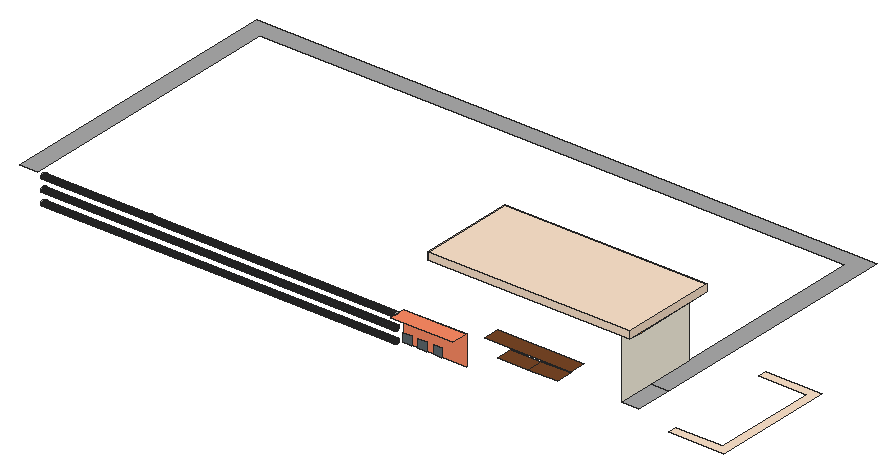
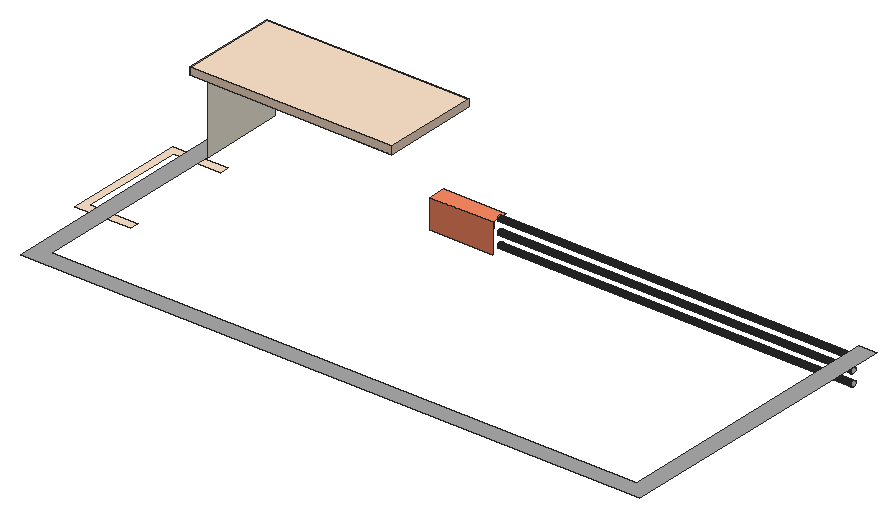
# SketchUp Ruby script. Lengths in inches.
U = 1.inch
M = Sketchup.active_model
def pt(a) = Geom::Point3d.new(a.map { |v| v * U })
def face(e, loops, mat)
  f = e.add_face(loops[0].map { |a| pt(a) })
  loops[1..].each { |l| e.add_face(l.map { |a| pt(a) }).erase! }
  f.material = f.back_material = mat if mat
  f
end
# faces: each face lists its corners as indices into pts; further lists are holes
def faces(e, pts, list, mat = nil) = list.each { |f| face(e, (f[0].is_a?(Array) ? f : [f]).map { |l| l.map { |i| pts[i] } }, mat) }
# xy, xz, yz: faces in a plane at the given z, y or x. An outline is a flat list of corners, or four numbers for a rectangle; further outlines are holes
def ring(l) = l.size == 4 ? [[l[0], l[1]], [l[2], l[1]], [l[2], l[3]], [l[0], l[3]]] : l.each_slice(2).to_a
def flat(e, list, mat, &to3) = list.each { |f| face(e, (f[0].is_a?(Array) ? f : [f]).map { |l| ring(l).map { |u, v| to3.(u, v) } }, mat) }
def xy(e, z, list, mat = nil) = flat(e, list, mat) { |x, y| [x, y, z] }
def xz(e, y, list, mat = nil) = flat(e, list, mat) { |x, z| [x, y, z] }
def yz(e, x, list, mat = nil) = flat(e, list, mat) { |y, z| [x, y, z] }
def lines(e, pts, list) = list.each { |a, b| e.add_line(pt(pts[a]), pt(pts[b])) }
# prism: a flat outline (further loops are holes) pulled along v
def prism(e, loops, v, mat = nil)
  f = face(e, loops, mat); d = Geom::Vector3d.new(v.map { |x| x * U })
  f.pushpull(f.normal.samedirection?(d) ? d.length : -d.length)
end
def box(e, o, s, mat = nil) = prism(e, [[o, [o[0] + s[0], o[1], o[2]], [o[0] + s[0], o[1] + s[1], o[2]], [o[0], o[1] + s[1], o[2]]]], [0, 0, s[2]], mat)
def at(x, y, z, deg = 0) = Geom::Transformation.translation(pt([x, y, z])) * Geom::Transformation.rotation(ORIGIN, Z_AXIS, deg.degrees)
def axes(o, x, y, z) = Geom::Transformation.new([*x, 0, *y, 0, *z, 0, *pt(o).to_a, 1])
def part(name) = M.definitions.add(name)
# library, detail: a bought-in or finely detailed component or shape, given as its bounding box
def library(name, o, s) = part(name).tap { |d| box(d.entities, o, s) }
def detail(e, o, s) = box(e.add_group.entities, o, s)
def put(e, d, t, mat = nil) = e.add_instance(d, t).tap { |i| i.material = mat if mat }
def group(e, t, mat = nil) = e.add_group.tap { |g| g.transformation = t; g.material = mat if mat }.entities
root = M.entities
M.materials.add("[Color B03]").color = [255, 140, 101]
M.materials.add("[Color C01]1").color = [255, 229, 204]
M.materials.add("[Color M03]").color = [170, 170, 170]
M.materials.add("[Formica Graystone]1").color = [255, 249, 231]
M.materials.add("[Formica Laminate Dark]").color = [50, 53, 60]
M.materials.add("[Formica Speckled Grey]").color = [94, 105, 111]
M.materials.add("[Wood Bamboo]").color = [177, 105, 43]
M.materials.add("[Wood Veneer 01]").color = [120, 70, 37]
xy(root,1017.818,[[1713.027,219.809,1866.152,219.809,1866.152,557.621,1713.027,557.621,1713.027,533.576,1844.714,533.576,1844.714,243.888,1713.027,243.888]],"[Color C01]1")
xy(root,1099.25,[[147.908,137.16,149.591,137.382,151.158,138.031,152.504,139.064,153.537,140.41,154.187,141.978,154.408,143.66,154.187,145.343,153.537,146.91,152.504,148.257,151.158,149.289,149.591,149.939,147.908,150.16,146.226,149.939,144.658,149.289,143.312,148.257,142.279,146.91,141.63,145.343,141.408,143.66,141.63,141.978,142.279,140.41,143.312,139.064,144.658,138.031,146.226,137.382]])
xy(root,1100.625,[[582.033,137.16,583.716,137.382,585.283,138.031,586.629,139.064,587.662,140.41,588.312,141.978,588.533,143.66,588.312,145.343,587.662,146.91,586.629,148.257,585.283,149.289,583.716,149.939,582.033,150.16,580.351,149.939,578.783,149.289,577.437,148.257,576.404,146.91,575.755,145.343,575.533,143.66,575.755,141.978,576.404,140.41,577.437,139.064,578.783,138.031,580.351,137.382]])
xy(root,1101.75,[[797.721,137.16,799.403,137.382,800.971,138.031,802.317,139.064,803.35,140.41,803.999,141.978,804.221,143.66,803.999,145.343,803.35,146.91,802.317,148.257,800.971,149.289,799.403,149.939,797.721,150.16,796.038,149.939,794.471,149.289,793.125,148.257,792.092,146.91,791.442,145.343,791.221,143.66,791.442,141.978,792.092,140.41,793.125,139.064,794.471,138.031,796.038,137.382],[984.137,138.709,985.819,138.93,987.387,139.58,988.733,140.613,989.766,141.959,990.416,143.527,990.637,145.209,990.416,146.891,989.766,148.459,988.733,149.805,987.387,150.838,985.819,151.487,984.137,151.709,982.455,151.487,980.887,150.838,979.541,149.805,978.508,148.459,977.859,146.891,977.637,145.209,977.859,143.527,978.508,141.959,979.541,140.613,980.887,139.58,982.455,138.93]])
xy(root,1102.645,[[1025.893,119.173,1198.268,166.042]],"[Color B03]")
xy(root,1104.303,[[341.783,137.16,343.466,137.382,345.033,138.031,346.379,139.064,347.412,140.41,348.062,141.978,348.283,143.66,348.062,145.343,347.412,146.91,347.14,147.265,336.426,147.265,336.154,146.91,335.505,145.343,335.283,143.66,335.505,141.978,336.154,140.41,337.187,139.064,338.533,138.031,340.101,137.382],[336.426,147.265,347.14,147.265,346.379,148.257,345.033,149.289,343.466,149.939,341.783,150.16,340.101,149.939,338.533,149.289,337.187,148.257]])
xy(root,1119.0625,[[1665.331,119.173,1713.027,219.809],[0,122.542,47.696,122.542,47.696,890.389,1665.331,890.389,1665.331,219.809,1713.027,219.809,1713.027,938.085,0,938.085]],"[Color M03]")
xy(root,1139.823,[[1358.015,73.861,1440.68,119.173],[1440.68,73.861,1523.345,119.173]],"[Wood Veneer 01]")
xy(root,1175.689,[[1322.149,73.861,1559.211,119.173]],"[Wood Veneer 01]")
xy(root,1305.375,[[1170.509,105.516,1168.39,105.795,1166.415,106.613,1164.719,107.914,1163.418,109.61,1162.6,111.585,1162.321,113.704,1162.6,115.823,1163.418,117.798,1164.719,119.493,1166.415,120.794,1168.39,121.612,1170.509,121.891,1172.628,121.612,1174.603,120.794,1176.298,119.493,1177.599,117.798,1178.417,115.823,1178.696,113.704,1178.417,111.585,1177.599,109.61,1176.298,107.914,1174.603,106.613,1172.628,105.795],[1198.268,119.173,1665.331,351.292],[1170.509,146.891,1168.39,147.17,1166.415,147.988,1164.719,149.289,1163.418,150.985,1162.6,152.96,1162.321,155.079,1162.6,157.198,1163.418,159.173,1164.719,160.868,1166.415,162.169,1168.39,162.987,1170.509,163.266,1172.628,162.987,1174.603,162.169,1176.298,160.868,1177.599,159.173,1178.417,157.198,1178.696,155.079,1178.417,152.96,1177.599,150.985,1176.298,149.289,1174.603,147.988,1172.628,147.17],[1170.509,209.204,1168.39,209.483,1166.415,210.301,1164.719,211.602,1163.418,213.298,1162.6,215.272,1162.321,217.391,1162.6,219.51,1163.418,221.485,1164.719,223.181,1166.415,224.482,1168.39,225.3,1170.509,225.579,1172.628,225.3,1174.603,224.482,1176.298,223.181,1177.599,221.485,1178.417,219.51,1178.696,217.391,1178.417,215.272,1177.599,213.298,1176.298,211.602,1174.603,210.301,1172.628,209.483],[1170.509,273.891,1168.39,274.17,1166.415,274.988,1164.719,276.289,1163.418,277.985,1162.6,279.96,1162.321,282.079,1162.6,284.198,1163.418,286.173,1164.719,287.868,1166.415,289.169,1168.39,289.987,1170.509,290.266,1172.628,289.987,1174.603,289.169,1176.298,287.868,1177.599,286.173,1178.417,284.198,1178.696,282.079,1178.417,279.96,1177.599,277.985,1176.298,276.289,1174.603,274.988,1172.628,274.17],
  [1170.509,317.579,1168.39,317.858,1166.415,318.676,1164.719,319.977,1163.418,321.673,1162.6,323.647,1162.321,325.766,1162.6,327.885,1163.418,329.86,1164.719,331.556,1166.415,332.857,1168.39,333.675,1170.509,333.954,1172.628,333.675,1174.603,332.857,1176.298,331.556,1177.599,329.86,1178.417,327.885,1178.696,325.766,1178.417,323.647,1177.599,321.673,1176.298,319.977,1174.603,318.676,1172.628,317.858]])
xy(root,1305.375,[[[1156.018,85.673,1156.018,351.292,1198.268,351.292,1198.268,119.173,1713.518,119.173,1713.518,85.673],[1170.509,105.516,1172.628,105.795,1174.603,106.613,1176.298,107.914,1177.599,109.61,1178.417,111.585,1178.696,113.704,1178.417,115.823,1177.599,117.798,1176.298,119.493,1174.603,120.794,1172.628,121.612,1170.509,121.891,1168.39,121.612,1166.415,120.794,1164.719,119.493,1163.418,117.798,1162.6,115.823,1162.321,113.704,1162.6,111.585,1163.418,109.61,1164.719,107.914,1166.415,106.613,1168.39,105.795],[1170.509,317.579,1172.628,317.858,1174.603,318.676,1176.298,319.977,1177.599,321.673,1178.417,323.647,1178.696,325.766,1178.417,327.885,1177.599,329.86,1176.298,331.556,1174.603,332.857,1172.628,333.675,1170.509,333.954,1168.39,333.675,1166.415,332.857,1164.719,331.556,1163.418,329.86,1162.6,327.885,1162.321,325.766,1162.6,323.647,1163.418,321.673,1164.719,319.977,1166.415,318.676,1168.39,317.858],[1170.509,146.891,1172.628,147.17,1174.603,147.988,1176.298,149.289,1177.599,150.985,1178.417,152.96,1178.696,155.079,1178.417,157.198,1177.599,159.173,1176.298,160.868,1174.603,162.169,1172.628,162.987,1170.509,163.266,1168.39,162.987,1166.415,162.169,1164.719,160.868,1163.418,159.173,1162.6,157.198,1162.321,155.079,1162.6,152.96,1163.418,150.985,1164.719,149.289,1166.415,147.988,1168.39,147.17],[1170.509,273.891,1172.628,274.17,1174.603,274.988,1176.298,276.289,1177.599,277.985,1178.417,279.96,1178.696,282.079,1178.417,284.198,1177.599,286.173,1176.298,287.868,1174.603,289.169,1172.628,289.987,1170.509,290.266,1168.39,289.987,1166.415,289.169,1164.719,287.868,1163.418,286.173,1162.6,284.198,1162.321,282.079,1162.6,279.96,1163.418,277.985,1164.719,276.289,1166.415,274.988,1168.39,274.17],[1170.509,209.204,1172.628,209.483,1174.603,210.301,1176.298,211.602,1177.599,213.298,1178.417,215.272,1178.696,217.391,1178.417,219.51,1177.599,221.485,1176.298,223.181,1174.603,224.482,1172.628,225.3,1170.509,225.579,1168.39,225.3,1166.415,224.482,1164.719,223.181,1163.418,221.485,1162.6,219.51,1162.321,217.391,1162.6,215.272,1163.418,213.298,1164.719,211.602,1166.415,210.301,1168.39,209.483]],[1665.331,119.173,1713.518,351.292]],"[Wood Bamboo]")
xy(root,1325.75,[[1156.018,85.673,1713.518,351.292]],"[Color C01]1")
xz(root,85.673,[[1156.018,1305.375,1713.518,1325.75]],"[Color C01]1")
xz(root,119.173,[[1060.122,1053.817,1083.872,1077.567],[1102.122,1053.817,1125.872,1077.567],[1144.684,1053.817,1168.434,1077.567]],"[Formica Speckled Grey]")
xz(root,166.042,[[1025.893,1021.906,1198.268,1102.645]],"[Color B03]")
xz(root,351.292,[[1156.018,1305.375,1713.518,1325.75]],"[Color C01]1")
yz(root,47.696,[[141.311,1027.741,139.531,1027.975,137.873,1028.662,136.449,1029.754,135.357,1031.178,134.67,1032.836,134.436,1034.616,134.67,1036.395,135.357,1038.053,136.449,1039.477,137.873,1040.57,139.531,1041.256,141.311,1041.491,143.09,1041.256,144.748,1040.57,146.172,1039.477,147.265,1038.053,147.952,1036.395,148.186,1034.616,147.952,1032.836,147.265,1031.178,146.172,1029.754,144.748,1028.662,143.09,1027.975],[141.311,1060.553,139.531,1060.787,137.873,1061.474,136.449,1062.567,135.357,1063.991,134.67,1065.649,134.436,1067.428,134.67,1069.208,135.357,1070.866,136.449,1072.29,137.873,1073.382,139.531,1074.069,141.311,1074.303,143.09,1074.069,144.748,1073.382,146.172,1072.29,147.265,1070.866,147.952,1069.208,148.186,1067.428,147.952,1065.649,147.265,1063.991,146.172,1062.567,144.748,1061.474,143.09,1060.787],[141.311,1093.991,139.531,1094.225,137.873,1094.912,136.449,1096.004,135.357,1097.428,134.67,1099.086,134.436,1100.866,134.67,1102.645,135.357,1104.303,136.449,1105.727,137.873,1106.82,139.531,1107.506,141.311,1107.741,143.09,1107.506,144.748,1106.82,146.172,1105.727,147.265,1104.303,147.952,1102.645,148.186,1100.866,147.952,1099.086,147.265,1097.428,146.172,1096.004,144.748,1094.912,143.09,1094.225]])
yz(root,1025.893,[[141.311,1093.991,143.09,1094.225,144.748,1094.912,146.172,1096.004,147.265,1097.428,147.952,1099.086,147.952,1102.645,134.67,1102.645,134.669,1102.638,134.669,1099.094,134.67,1099.086,135.357,1097.428,136.449,1096.004,137.873,1094.912,139.531,1094.225],[134.669,1099.094,134.436,1100.866,134.669,1102.638],[147.952,1099.094,147.952,1102.638,148.186,1100.866],[134.67,1102.645,147.952,1102.645,147.265,1104.303,146.172,1105.727,144.748,1106.82,143.09,1107.506,141.311,1107.741,139.531,1107.506,137.873,1106.82,136.449,1105.727,135.357,1104.303]])
yz(root,1156.018,[[85.673,1305.375,351.292,1325.75]],"[Color C01]1")
yz(root,1665.331,[[119.173,1119.0625,351.292,1305.375]],"[Formica Graystone]1")
yz(root,1713.518,[[85.673,1305.375,351.292,1325.75]],"[Color C01]1")
p = [[47.696,139.531,1027.975],[47.696,141.311,1027.741],[1025.893,141.311,1027.741],[1025.893,139.531,1027.975],[47.696,143.09,1027.975],[1025.893,143.09,1027.975],
  [47.696,137.873,1028.662],[1025.893,137.873,1028.662],[47.696,144.748,1028.662],[1025.893,144.748,1028.662],[47.696,136.449,1029.754],[1025.893,136.449,1029.754],
  [47.696,146.172,1029.754],[1025.893,146.172,1029.754],[47.696,135.357,1031.178],[1025.893,135.357,1031.178],[47.696,147.265,1031.178],[1025.893,147.265,1031.178],
  [47.696,134.67,1032.836],[1025.893,134.67,1032.836],[47.696,147.952,1032.836],[1025.893,147.952,1032.836],[47.696,134.436,1034.616],[1025.893,134.436,1034.616],
  [47.696,148.186,1034.616],[1025.893,148.186,1034.616],[47.696,134.67,1036.395],[1025.893,134.67,1036.395],[47.696,147.952,1036.395],[1025.893,147.952,1036.395],
  [47.696,135.357,1038.053],[1025.893,135.357,1038.053],[47.696,147.265,1038.053],[1025.893,147.265,1038.053],[47.696,136.449,1039.477],[1025.893,136.449,1039.477],
  [47.696,146.172,1039.477],[1025.893,146.172,1039.477],[47.696,137.873,1040.57],[1025.893,137.873,1040.57],[47.696,144.748,1040.57],[1025.893,144.748,1040.57],
  [47.696,139.531,1041.256],[1025.893,139.531,1041.256],[47.696,143.09,1041.256],[1025.893,143.09,1041.256],[47.696,141.311,1041.491],[1025.893,141.311,1041.491],
  [47.696,139.531,1060.787],[47.696,141.311,1060.553],[1025.893,141.311,1060.553],[1025.893,139.531,1060.787],[47.696,143.09,1060.787],[1025.893,143.09,1060.787],
  [47.696,137.873,1061.474],[1025.893,137.873,1061.474],[47.696,144.748,1061.474],[1025.893,144.748,1061.474],[47.696,136.449,1062.567],[1025.893,136.449,1062.567],
  [47.696,146.172,1062.567],[1025.893,146.172,1062.567],[47.696,135.357,1063.991],[1025.893,135.357,1063.991],[47.696,147.265,1063.991],[1025.893,147.265,1063.991],
  [47.696,134.67,1065.649],[1025.893,134.67,1065.649],[47.696,147.952,1065.649],[1025.893,147.952,1065.649],[47.696,134.436,1067.428],[1025.893,134.436,1067.428],
  [47.696,148.186,1067.428],[1025.893,148.186,1067.428],[47.696,134.67,1069.208],[1025.893,134.67,1069.208],[47.696,147.952,1069.208],[1025.893,147.952,1069.208],
  [47.696,135.357,1070.866],[1025.893,135.357,1070.866],[47.696,147.265,1070.866],[1025.893,147.265,1070.866],[47.696,136.449,1072.29],[1025.893,136.449,1072.29],
  [47.696,146.172,1072.29],[1025.893,146.172,1072.29],[47.696,137.873,1073.382],[1025.893,137.873,1073.382],[47.696,144.748,1073.382],[1025.893,144.748,1073.382],
  [47.696,139.531,1074.069],[1025.893,139.531,1074.069],[47.696,143.09,1074.069],[1025.893,143.09,1074.069],[47.696,141.311,1074.303],[1025.893,141.311,1074.303],
  [47.696,139.531,1094.225],[47.696,141.311,1093.991],[1025.893,141.311,1093.991],[1025.893,139.531,1094.225],[47.696,143.09,1094.225],[1025.893,143.09,1094.225],
  [47.696,137.873,1094.912],[1025.893,137.873,1094.912],[47.696,144.748,1094.912],[1025.893,144.748,1094.912],[47.696,136.449,1096.004],[1025.893,136.449,1096.004],
  [47.696,146.172,1096.004],[1025.893,146.172,1096.004],[47.696,135.357,1097.428],[1025.893,135.357,1097.428],[47.696,147.265,1097.428],[1025.893,147.265,1097.428],
  [47.696,134.67,1099.086],[1025.893,134.67,1099.086],[47.696,147.952,1099.086],[1025.893,147.952,1099.086],[47.696,134.436,1100.866],[1025.893,134.669,1099.094],
  [1025.893,134.436,1100.866],[47.696,148.186,1100.866],[1025.893,148.186,1100.866],[1025.893,147.952,1099.094],[47.696,134.67,1102.645],[1025.893,134.669,1102.638],
  [1025.893,134.67,1102.645],[47.696,147.952,1102.645],[1025.893,147.952,1102.645],[1025.893,147.952,1102.638],[47.696,135.357,1104.303],[1025.893,135.357,1104.303],
  [47.696,147.265,1104.303],[336.426,147.265,1104.303],[347.14,147.265,1104.303],[1025.893,147.265,1104.303],[47.696,136.449,1105.727],[1025.893,136.449,1105.727],
  [47.696,146.172,1105.727],[1025.893,146.172,1105.727],[47.696,137.873,1106.82],[1025.893,137.873,1106.82],[47.696,144.748,1106.82],[1025.893,144.748,1106.82],
  [47.696,139.531,1107.506],[1025.893,139.531,1107.506],[47.696,143.09,1107.506],[1025.893,143.09,1107.506],[47.696,141.311,1107.741],[1025.893,141.311,1107.741]]
faces(root,p,[[0,1,2,3],[1,4,5,2],[6,0,3,7],[4,8,9,5],[10,6,7,11],[8,12,13,9],[14,10,11,15],[12,16,17,13],
  [18,14,15,19],[16,20,21,17],[22,18,19,23],[20,24,25,21],[26,22,23,27],[24,28,29,25],[30,26,27,31],[28,32,33,29],
  [34,30,31,35],[32,36,37,33],[38,34,35,39],[36,40,41,37],[42,38,39,43],[40,44,45,41],[46,42,43,47],[44,46,47,45],
  [48,49,50,51],[49,52,53,50],[54,48,51,55],[52,56,57,53],[58,54,55,59],[56,60,61,57],[62,58,59,63],[60,64,65,61],
  [66,62,63,67],[64,68,69,65],[70,66,67,71],[68,72,73,69],[74,70,71,75],[72,76,77,73],[78,74,75,79],[76,80,81,77],
  [82,78,79,83],[80,84,85,81],[86,82,83,87],[84,88,89,85],[90,86,87,91],[88,92,93,89],[94,90,91,95],[92,94,95,93],
  [96,97,98,99],[97,100,101,98],[102,96,99,103],[100,104,105,101],[106,102,103,107],[104,108,109,105],[110,106,107,111],[108,112,113,109],
  [114,110,111,115],[112,116,117,113],[118,114,115,119,120],[116,121,122,123,117],[124,118,120,125,126],[121,127,128,129,122],[130,124,126,131],[127,132,133,134,135,128],
  [136,130,131,137],[132,138,139,135,134,133],[140,136,137,141],[138,142,143,139],[144,140,141,145],[142,146,147,143],[148,144,145,149],[146,148,149,147]],"[Formica Laminate Dark]")
